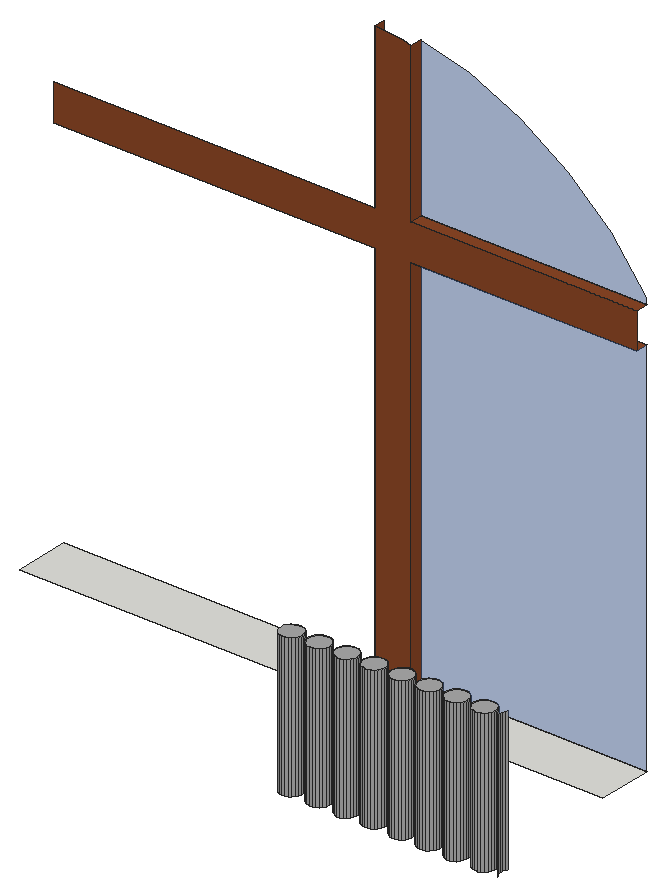
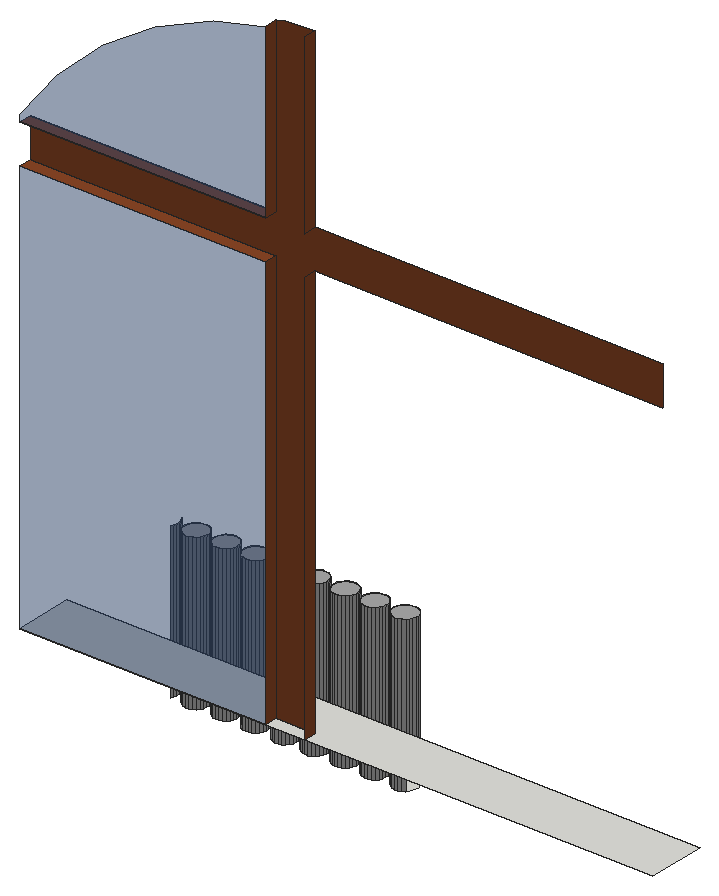
# SketchUp Ruby script. Lengths in inches.
U = 1.inch
M = Sketchup.active_model
def pt(a) = Geom::Point3d.new(a.map { |v| v * U })
def face(e, loops, mat)
  f = e.add_face(loops[0].map { |a| pt(a) })
  loops[1..].each { |l| e.add_face(l.map { |a| pt(a) }).erase! }
  f.material = f.back_material = mat if mat
  f
end
# faces: each face lists its corners as indices into pts; further lists are holes
def faces(e, pts, list, mat = nil) = list.each { |f| face(e, (f[0].is_a?(Array) ? f : [f]).map { |l| l.map { |i| pts[i] } }, mat) }
# xy, xz, yz: faces in a plane at the given z, y or x. An outline is a flat list of corners, or four numbers for a rectangle; further outlines are holes
def ring(l) = l.size == 4 ? [[l[0], l[1]], [l[2], l[1]], [l[2], l[3]], [l[0], l[3]]] : l.each_slice(2).to_a
def flat(e, list, mat, &to3) = list.each { |f| face(e, (f[0].is_a?(Array) ? f : [f]).map { |l| ring(l).map { |u, v| to3.(u, v) } }, mat) }
def xy(e, z, list, mat = nil) = flat(e, list, mat) { |x, y| [x, y, z] }
def xz(e, y, list, mat = nil) = flat(e, list, mat) { |x, z| [x, y, z] }
def yz(e, x, list, mat = nil) = flat(e, list, mat) { |y, z| [x, y, z] }
def lines(e, pts, list) = list.each { |a, b| e.add_line(pt(pts[a]), pt(pts[b])) }
# prism: a flat outline (further loops are holes) pulled along v
def prism(e, loops, v, mat = nil)
  f = face(e, loops, mat); d = Geom::Vector3d.new(v.map { |x| x * U })
  f.pushpull(f.normal.samedirection?(d) ? d.length : -d.length)
end
def box(e, o, s, mat = nil) = prism(e, [[o, [o[0] + s[0], o[1], o[2]], [o[0] + s[0], o[1] + s[1], o[2]], [o[0], o[1] + s[1], o[2]]]], [0, 0, s[2]], mat)
def at(x, y, z, deg = 0) = Geom::Transformation.translation(pt([x, y, z])) * Geom::Transformation.rotation(ORIGIN, Z_AXIS, deg.degrees)
def axes(o, x, y, z) = Geom::Transformation.new([*x, 0, *y, 0, *z, 0, *pt(o).to_a, 1])
def part(name) = M.definitions.add(name)
# library, detail: a bought-in or finely detailed component or shape, given as its bounding box
def library(name, o, s) = part(name).tap { |d| box(d.entities, o, s) }
def detail(e, o, s) = box(e.add_group.entities, o, s)
def put(e, d, t, mat = nil) = e.add_instance(d, t).tap { |i| i.material = mat if mat }
def group(e, t, mat = nil) = e.add_group.tap { |g| g.transformation = t; g.material = mat if mat }.entities
root = M.entities
M.materials.add("[0042_Sienna]").color = [137, 70, 38]
M.materials.add("[0132_LightGray]").color = [169, 169, 169]
M.materials.add("[Translucent Glass Blue]").color = [66, 99, 158]
M.materials["[Translucent Glass Blue]"].alpha = 0.5
xy(root,336.85,[[302.77,32.1,302.31,32.2,301.89,32.42,301.54,32.73,301.28,33.13,301.13,33.58,301.11,34.05,301.2,34.52,301.42,34.9375,301.73,35.29,302.13,35.55,302.58,35.69,303.05,35.72,303.52,35.62,303.9375,35.41,304.29,35.09,304.55,34.69,304.69,34.24,304.72,33.77,304.62,33.31,304.41,32.89,304.09,32.53,303.69,32.28,303.24,32.13],[307.33,32.1,306.87,32.2,306.45,32.42,306.1,32.73,305.84,33.13,305.69,33.58,305.67,34.05,305.77,34.52,305.98,34.9375,306.3,35.29,306.69,35.55,307.14,35.69,307.62,35.72,308.08,35.62,308.5,35.41,308.85,35.09,309.11,34.69,309.26,34.24,309.28,33.77,309.18,33.31,308.97,32.89,308.65,32.53,308.26,32.28,307.81,32.13],[311.9,32.1,311.43,32.2,311.01,32.42,310.66,32.73,310.4,33.13,310.26,33.58,310.23,34.05,310.33,34.52,310.54,34.9375,310.86,35.29,311.26,35.55,311.71,35.69,312.18,35.72,312.64,35.62,313.0625,35.41,313.42,35.09,313.67,34.69,313.82,34.24,313.84,33.77,313.75,33.31,313.53,32.89,313.22,32.53,312.82,32.28,312.37,32.13],[316.46,32.1,316,32.2,315.57,32.42,315.22,32.73,314.97,33.13,314.82,33.58,314.79,34.05,314.89,34.52,315.11,34.9375,315.42,35.29,315.82,35.55,316.27,35.69,316.74,35.72,317.2,35.62,317.625,35.41,317.98,35.09,318.24,34.69,318.38,34.24,318.41,33.77,318.31,33.31,318.09,32.89,317.78,32.53,317.38,32.28,316.93,32.13],[321.02,32.1,320.56,32.2,320.14,32.42,319.79,32.73,319.53,33.13,319.38,33.58,319.36,34.05,319.45,34.52,319.67,34.9375,319.98,35.29,320.38,35.55,320.83,35.69,321.3,35.72,321.77,35.62,322.1875,35.41,322.54,35.09,322.8,34.69,322.94,34.24,322.97,33.77,322.87,33.31,322.66,32.89,322.34,32.53,321.94,32.28,321.49,32.13],
  [325.58,32.1,325.12,32.2,324.7,32.42,324.35,32.73,324.09,33.13,323.94,33.58,323.92,34.05,324.02,34.52,324.23,34.9375,324.55,35.29,324.94,35.55,325.39,35.69,325.87,35.72,326.33,35.62,326.75,35.41,327.1,35.09,327.36,34.69,327.51,34.24,327.53,33.77,327.43,33.31,327.22,32.89,326.9,32.53,326.51,32.28,326.06,32.13],[330.15,32.1,329.68,32.2,329.26,32.42,328.91,32.73,328.65,33.13,328.51,33.58,328.48,34.05,328.58,34.52,328.79,34.9375,329.11,35.29,329.51,35.55,329.96,35.69,330.43,35.72,330.89,35.62,331.3125,35.41,331.67,35.09,331.92,34.69,332.07,34.24,332.09,33.77,332,33.31,331.78,32.89,331.47,32.53,331.07,32.28,330.62,32.13],[334.71,32.1,334.25,32.2,333.82,32.42,333.47,32.73,333.22,33.13,333.07,33.58,333.04,34.05,333.14,34.52,333.36,34.9375,333.67,35.29,334.07,35.55,334.52,35.69,334.99,35.72,335.45,35.62,335.875,35.41,336.23,35.09,336.49,34.69,336.63,34.24,336.66,33.77,336.56,33.31,336.34,32.89,336.03,32.53,335.63,32.28,335.18,32.13]])
xy(root,348.85,[[252.45,40.6875,349.14,40.6875,349.14,49.6875,311.64,49.6875,311.64,47.6875,305.64,47.6875,305.64,49.6875,252.45,49.6875],[305.64,47.6875,311.64,49.6875]])
xy(root,360.41,[[302.77,32.1,303.24,32.13,303.69,32.28,304.09,32.53,304.41,32.89,304.62,33.31,304.72,33.77,304.69,34.24,304.55,34.69,304.29,35.09,303.9375,35.41,303.52,35.62,303.05,35.72,302.58,35.69,302.13,35.55,301.73,35.29,301.42,34.9375,301.2,34.52,301.11,34.05,301.13,33.58,301.28,33.13,301.54,32.73,301.89,32.42,302.31,32.2],[307.33,32.1,307.81,32.13,308.26,32.28,308.65,32.53,308.97,32.89,309.18,33.31,309.28,33.77,309.26,34.24,309.11,34.69,308.85,35.09,308.5,35.41,308.08,35.62,307.62,35.72,307.14,35.69,306.69,35.55,306.3,35.29,305.98,34.9375,305.77,34.52,305.67,34.05,305.69,33.58,305.84,33.13,306.1,32.73,306.45,32.42,306.87,32.2],[311.9,32.1,312.37,32.13,312.82,32.28,313.22,32.53,313.53,32.89,313.75,33.31,313.84,33.77,313.82,34.24,313.67,34.69,313.42,35.09,313.0625,35.41,312.64,35.62,312.18,35.72,311.71,35.69,311.26,35.55,310.86,35.29,310.54,34.9375,310.33,34.52,310.23,34.05,310.26,33.58,310.4,33.13,310.66,32.73,311.01,32.42,311.43,32.2],[316.46,32.1,316.93,32.13,317.38,32.28,317.78,32.53,318.09,32.89,318.31,33.31,318.41,33.77,318.38,34.24,318.24,34.69,317.98,35.09,317.625,35.41,317.2,35.62,316.74,35.72,316.27,35.69,315.82,35.55,315.42,35.29,315.11,34.9375,314.89,34.52,314.79,34.05,314.82,33.58,314.97,33.13,315.22,32.73,315.57,32.42,316,32.2],[321.02,32.1,321.49,32.13,321.94,32.28,322.34,32.53,322.66,32.89,322.87,33.31,322.97,33.77,322.94,34.24,322.8,34.69,322.54,35.09,322.1875,35.41,321.77,35.62,321.3,35.72,320.83,35.69,320.38,35.55,319.98,35.29,319.67,34.9375,319.45,34.52,319.36,34.05,319.38,33.58,319.53,33.13,319.79,32.73,320.14,32.42,320.56,32.2],
  [325.58,32.1,326.06,32.13,326.51,32.28,326.9,32.53,327.22,32.89,327.43,33.31,327.53,33.77,327.51,34.24,327.36,34.69,327.1,35.09,326.75,35.41,326.33,35.62,325.87,35.72,325.39,35.69,324.94,35.55,324.55,35.29,324.23,34.9375,324.02,34.52,323.92,34.05,323.94,33.58,324.09,33.13,324.35,32.73,324.7,32.42,325.12,32.2],[330.15,32.1,330.62,32.13,331.07,32.28,331.47,32.53,331.78,32.89,332,33.31,332.09,33.77,332.07,34.24,331.92,34.69,331.67,35.09,331.3125,35.41,330.89,35.62,330.43,35.72,329.96,35.69,329.51,35.55,329.11,35.29,328.79,34.9375,328.58,34.52,328.48,34.05,328.51,33.58,328.65,33.13,328.91,32.73,329.26,32.42,329.68,32.2],[334.71,32.1,335.18,32.13,335.63,32.28,336.03,32.53,336.34,32.89,336.56,33.31,336.66,33.77,336.63,34.24,336.49,34.69,336.23,35.09,335.875,35.41,335.45,35.62,334.99,35.72,334.52,35.69,334.07,35.55,333.67,35.29,333.36,34.9375,333.14,34.52,333.04,34.05,333.07,33.58,333.22,33.13,333.47,32.73,333.82,32.42,334.25,32.2]],"[0132_LightGray]")
xy(root,412.18,[[311.64,47.6875,349.14,49.6875]],"[0042_Sienna]")
xy(root,418.18,[[311.64,47.6875,349.14,49.6875]],"[0042_Sienna]")
xz(root,47.6875,[[305.64,348.85,311.64,348.85,311.64,412.18,349.14,412.18,349.14,418.18,311.64,418.18,311.64,444.4,310.32,444.74,305.64,445.13,305.64,418.18,252.45,418.18,252.45,412.18,305.64,412.18]],"[0042_Sienna]")
xz(root,49.6875,[[311.64,348.85,349.14,412.18],[311.64,418.18,349.14,418.18,349.14,419.18,343.31,426.75,336.3,433.26,328.32,438.52,319.58,442.38,311.64,444.4]],"[Translucent Glass Blue]")
yz(root,305.64,[[47.6875,348.85,49.6875,412.18],[47.6875,418.18,49.6875,445.13]],"[0042_Sienna]")
yz(root,311.64,[[47.6875,348.85,49.6875,412.18],[47.6875,418.18,49.6875,444.4]],"[0042_Sienna]")
p = [[302.31,32.2,336.85],[302.77,32.1,336.85],[302.77,32.1,360.41],[302.31,32.2,360.41],[303.24,32.13,336.85],[303.24,32.13,360.41],
  [303.69,32.28,336.85],[303.69,32.28,360.41],[306.87,32.2,336.85],[307.33,32.1,336.85],[307.33,32.1,360.41],[306.87,32.2,360.41],
  [307.81,32.13,336.85],[307.81,32.13,360.41],[308.26,32.28,336.85],[308.26,32.28,360.41],[311.43,32.2,336.85],[311.9,32.1,336.85],
  [311.9,32.1,360.41],[311.43,32.2,360.41],[312.37,32.13,336.85],[312.37,32.13,360.41],[312.82,32.28,336.85],[312.82,32.28,360.41],
  [316,32.2,336.85],[316.46,32.1,336.85],[316.46,32.1,360.41],[316,32.2,360.41],[316.93,32.13,336.85],[316.93,32.13,360.41],
  [317.38,32.28,336.85],[317.38,32.28,360.41],[320.56,32.2,336.85],[321.02,32.1,336.85],[321.02,32.1,360.41],[320.56,32.2,360.41],
  [321.49,32.13,336.85],[321.49,32.13,360.41],[321.94,32.28,336.85],[321.94,32.28,360.41],[325.12,32.2,336.85],[325.58,32.1,336.85],
  [325.58,32.1,360.41],[325.12,32.2,360.41],[326.06,32.13,336.85],[326.06,32.13,360.41],[326.51,32.28,336.85],[326.51,32.28,360.41],
  [329.68,32.2,336.85],[330.15,32.1,336.85],[330.15,32.1,360.41],[329.68,32.2,360.41],[330.62,32.13,336.85],[330.62,32.13,360.41],
  [331.07,32.28,336.85],[331.07,32.28,360.41],[334.25,32.2,336.85],[334.71,32.1,336.85],[334.71,32.1,360.41],[334.25,32.2,360.41],
  [335.18,32.13,336.85],[335.18,32.13,360.41],[335.63,32.28,336.85],[335.63,32.28,360.41],[301.89,32.42,336.85],[301.89,32.42,360.41],
  [306.45,32.42,336.85],[306.45,32.42,360.41],[311.01,32.42,336.85],[311.01,32.42,360.41],[315.57,32.42,336.85],[315.57,32.42,360.41],
  [320.14,32.42,336.85],[320.14,32.42,360.41],[324.7,32.42,336.85],[324.7,32.42,360.41],[329.26,32.42,336.85],[329.26,32.42,360.41],
  [333.82,32.42,336.85],[333.82,32.42,360.41],[304.09,32.53,336.85],[304.09,32.53,360.41],[308.65,32.53,336.85],[308.65,32.53,360.41],
  [313.22,32.53,336.85],[313.22,32.53,360.41],[317.78,32.53,336.85],[317.78,32.53,360.41],[322.34,32.53,336.85],[322.34,32.53,360.41],
  [326.9,32.53,336.85],[326.9,32.53,360.41],[331.47,32.53,336.85],[331.47,32.53,360.41],[336.03,32.53,336.85],[336.03,32.53,360.41],
  [301.54,32.73,336.85],[301.54,32.73,360.41],[306.1,32.73,336.85],[306.1,32.73,360.41],[310.66,32.73,336.85],[310.66,32.73,360.41],
  [315.22,32.73,336.85],[315.22,32.73,360.41],[319.79,32.73,336.85],[319.79,32.73,360.41],[324.35,32.73,336.85],[324.35,32.73,360.41],
  [328.91,32.73,336.85],[328.91,32.73,360.41],[333.47,32.73,336.85],[333.47,32.73,360.41],[304.41,32.89,336.85],[304.41,32.89,360.41],
  [308.97,32.89,336.85],[308.97,32.89,360.41],[313.53,32.89,336.85],[313.53,32.89,360.41],[318.09,32.89,336.85],[318.09,32.89,360.41],
  [322.66,32.89,336.85],[322.66,32.89,360.41],[327.22,32.89,336.85],[327.22,32.89,360.41],[331.78,32.89,336.85],[331.78,32.89,360.41],
  [336.34,32.89,336.85],[336.34,32.89,360.41],[305.84,33.13,336.85],[305.84,33.13,360.41],[310.4,33.13,336.85],[310.4,33.13,360.41],
  [314.97,33.13,336.85],[314.97,33.13,360.41],[319.53,33.13,336.85],[319.53,33.13,360.41],[324.09,33.13,336.85],[324.09,33.13,360.41],
  [328.65,33.13,336.85],[328.65,33.13,360.41],[333.22,33.13,336.85],[333.22,33.13,360.41],[337.78,33.13,336.85],[338.04,32.73,336.85],
  [338.04,32.73,360.41],[337.78,33.13,360.41],[304.62,33.31,336.85],[304.62,33.31,360.41],[309.18,33.31,336.85],[309.18,33.31,360.41],
  [313.75,33.31,336.85],[313.75,33.31,360.41],[318.31,33.31,336.85],[318.31,33.31,360.41],[322.87,33.31,336.85],[322.87,33.31,360.41],
  [327.43,33.31,336.85],[327.43,33.31,360.41],[332,33.31,336.85],[332,33.31,360.41],[336.56,33.31,336.85],[336.56,33.31,360.41],
  [305.69,33.58,336.85],[305.69,33.58,360.41],[310.26,33.58,336.85],[310.26,33.58,360.41],[314.82,33.58,336.85],[314.82,33.58,360.41],
  [319.38,33.58,336.85],[319.38,33.58,360.41],[323.94,33.58,336.85],[323.94,33.58,360.41],[328.51,33.58,336.85],[328.51,33.58,360.41],
  [333.07,33.58,336.85],[333.07,33.58,360.41],[337.63,33.58,336.85],[337.63,33.58,360.41],[304.72,33.77,336.85],[304.72,33.77,360.41],
  [309.28,33.77,336.85],[309.28,33.77,360.41],[313.84,33.77,336.85],[313.84,33.77,360.41],[318.41,33.77,336.85],[318.41,33.77,360.41],
  [322.97,33.77,336.85],[322.97,33.77,360.41],[327.53,33.77,336.85],[327.53,33.77,360.41],[332.09,33.77,336.85],[332.09,33.77,360.41],
  [336.66,33.77,336.85],[336.66,33.77,360.41],[305.67,34.05,336.85],[305.67,34.05,360.41],[310.23,34.05,336.85],[310.23,34.05,360.41],
  [314.79,34.05,336.85],[314.79,34.05,360.41],[319.36,34.05,336.85],[319.36,34.05,360.41],[323.92,34.05,336.85],[323.92,34.05,360.41],
  [328.48,34.05,336.85],[328.48,34.05,360.41],[333.04,34.05,336.85],[333.04,34.05,360.41],[337.61,34.05,336.85],[337.61,34.05,360.41],
  [304.69,34.24,336.85],[304.69,34.24,360.41],[309.26,34.24,336.85],[309.26,34.24,360.41],[313.82,34.24,336.85],[313.82,34.24,360.41],
  [318.38,34.24,336.85],[318.38,34.24,360.41],[322.94,34.24,336.85],[322.94,34.24,360.41],[327.51,34.24,336.85],[327.51,34.24,360.41],
  [332.07,34.24,336.85],[332.07,34.24,360.41],[336.63,34.24,336.85],[336.63,34.24,360.41],[305.77,34.52,336.85],[305.77,34.52,360.41],
  [310.33,34.52,336.85],[310.33,34.52,360.41],[314.89,34.52,336.85],[314.89,34.52,360.41],[319.45,34.52,336.85],[319.45,34.52,360.41],
  [324.02,34.52,336.85],[324.02,34.52,360.41],[328.58,34.52,336.85],[328.58,34.52,360.41],[333.14,34.52,336.85],[333.14,34.52,360.41],
  [337.7,34.52,336.85],[337.7,34.52,360.41],[304.55,34.69,336.85],[304.55,34.69,360.41],[309.11,34.69,336.85],[309.11,34.69,360.41],
  [313.67,34.69,336.85],[313.67,34.69,360.41],[318.24,34.69,336.85],[318.24,34.69,360.41],[322.8,34.69,336.85],[322.8,34.69,360.41],
  [327.36,34.69,336.85],[327.36,34.69,360.41],[331.92,34.69,336.85],[331.92,34.69,360.41],[336.49,34.69,336.85],[336.49,34.69,360.41],
  [305.98,34.9375,336.85],[305.98,34.9375,360.41],[310.54,34.9375,336.85],[310.54,34.9375,360.41],[315.11,34.9375,336.85],[315.11,34.9375,360.41],
  [319.67,34.9375,336.85],[319.67,34.9375,360.41],[324.23,34.9375,336.85],[324.23,34.9375,360.41],[328.79,34.9375,336.85],[328.79,34.9375,360.41],
  [333.36,34.9375,336.85],[333.36,34.9375,360.41],[337.92,34.9375,336.85],[337.92,34.9375,360.41],[304.29,35.09,336.85],[304.29,35.09,360.41],
  [308.85,35.09,336.85],[308.85,35.09,360.41],[313.42,35.09,336.85],[313.42,35.09,360.41],[317.98,35.09,336.85],[317.98,35.09,360.41],
  [322.54,35.09,336.85],[322.54,35.09,360.41],[327.1,35.09,336.85],[327.1,35.09,360.41],[331.67,35.09,336.85],[331.67,35.09,360.41],
  [336.23,35.09,336.85],[336.23,35.09,360.41],[306.3,35.29,336.85],[306.3,35.29,360.41],[310.86,35.29,336.85],[310.86,35.29,360.41],
  [315.42,35.29,336.85],[315.42,35.29,360.41],[319.98,35.29,336.85],[319.98,35.29,360.41],[324.55,35.29,336.85],[324.55,35.29,360.41],
  [329.11,35.29,336.85],[329.11,35.29,360.41],[333.67,35.29,336.85],[333.67,35.29,360.41],[303.9375,35.41,336.85],[303.9375,35.41,360.41],
  [308.5,35.41,336.85],[308.5,35.41,360.41],[313.0625,35.41,336.85],[313.0625,35.41,360.41],[317.625,35.41,336.85],[317.625,35.41,360.41],
  [322.1875,35.41,336.85],[322.1875,35.41,360.41],[326.75,35.41,336.85],[326.75,35.41,360.41],[331.3125,35.41,336.85],[331.3125,35.41,360.41],
  [335.875,35.41,336.85],[335.875,35.41,360.41],[302.13,35.55,336.85],[301.73,35.29,336.85],[301.73,35.29,360.41],[302.13,35.55,360.41],
  [306.69,35.55,336.85],[306.69,35.55,360.41],[311.26,35.55,336.85],[311.26,35.55,360.41],[315.82,35.55,336.85],[315.82,35.55,360.41],
  [320.38,35.55,336.85],[320.38,35.55,360.41],[324.94,35.55,336.85],[324.94,35.55,360.41],[329.51,35.55,336.85],[329.51,35.55,360.41],
  [334.07,35.55,336.85],[334.07,35.55,360.41],[303.52,35.62,336.85],[303.52,35.62,360.41],[308.08,35.62,336.85],[308.08,35.62,360.41],
  [312.64,35.62,336.85],[312.64,35.62,360.41],[317.2,35.62,336.85],[317.2,35.62,360.41],[321.77,35.62,336.85],[321.77,35.62,360.41],
  [326.33,35.62,336.85],[326.33,35.62,360.41],[330.89,35.62,336.85],[330.89,35.62,360.41],[335.45,35.62,336.85],[335.45,35.62,360.41],
  [302.58,35.69,336.85],[302.58,35.69,360.41],[307.14,35.69,336.85],[307.14,35.69,360.41],[311.71,35.69,336.85],[311.71,35.69,360.41],
  [316.27,35.69,336.85],[316.27,35.69,360.41],[320.83,35.69,336.85],[320.83,35.69,360.41],[325.39,35.69,336.85],[325.39,35.69,360.41],
  [329.96,35.69,336.85],[329.96,35.69,360.41],[334.52,35.69,336.85],[334.52,35.69,360.41],[303.05,35.72,336.85],[303.05,35.72,360.41],
  [307.62,35.72,336.85],[307.62,35.72,360.41],[312.18,35.72,336.85],[312.18,35.72,360.41],[316.74,35.72,336.85],[316.74,35.72,360.41],
  [321.3,35.72,336.85],[321.3,35.72,360.41],[325.87,35.72,336.85],[325.87,35.72,360.41],[330.43,35.72,336.85],[330.43,35.72,360.41],
  [334.99,35.72,336.85],[334.99,35.72,360.41]]
faces(root,p,[[0,1,2,3],[1,4,5,2],[4,6,7,5],[8,9,10,11],[9,12,13,10],[12,14,15,13],[16,17,18,19],[17,20,21,18],
  [20,22,23,21],[24,25,26,27],[25,28,29,26],[28,30,31,29],[32,33,34,35],[33,36,37,34],[36,38,39,37],[40,41,42,43],
  [41,44,45,42],[44,46,47,45],[48,49,50,51],[49,52,53,50],[52,54,55,53],[56,57,58,59],[57,60,61,58],[60,62,63,61],
  [64,0,3,65],[66,8,11,67],[68,16,19,69],[70,24,27,71],[72,32,35,73],[74,40,43,75],[76,48,51,77],[78,56,59,79],
  [6,80,81,7],[14,82,83,15],[22,84,85,23],[30,86,87,31],[38,88,89,39],[46,90,91,47],[54,92,93,55],[62,94,95,63],
  [96,64,65,97],[98,66,67,99],[100,68,69,101],[102,70,71,103],[104,72,73,105],[106,74,75,107],[108,76,77,109],[110,78,79,111],
  [80,112,113,81],[82,114,115,83],[84,116,117,85],[86,118,119,87],[88,120,121,89],[90,122,123,91],[92,124,125,93],[94,126,127,95],
  [128,98,99,129],[130,100,101,131],[132,102,103,133],[134,104,105,135],[136,106,107,137],[138,108,109,139],[140,110,111,141],[142,143,144,145],
  [112,146,147,113],[114,148,149,115],[116,150,151,117],[118,152,153,119],[120,154,155,121],[122,156,157,123],[124,158,159,125],[126,160,161,127],
  [162,128,129,163],[164,130,131,165],[166,132,133,167],[168,134,135,169],[170,136,137,171],[172,138,139,173],[174,140,141,175],[176,142,145,177],
  [146,178,179,147],[148,180,181,149],[150,182,183,151],[152,184,185,153],[154,186,187,155],[156,188,189,157],[158,190,191,159],[160,192,193,161],
  [194,162,163,195],[196,164,165,197],[198,166,167,199],[200,168,169,201],[202,170,171,203],[204,172,173,205],[206,174,175,207],[208,176,177,209],
  [178,210,211,179],[180,212,213,181],[182,214,215,183],[184,216,217,185],[186,218,219,187],[188,220,221,189],[190,222,223,191],[192,224,225,193],
  [226,194,195,227],[228,196,197,229],[230,198,199,231],[232,200,201,233],[234,202,203,235],[236,204,205,237],[238,206,207,239],[240,208,209,241],
  [210,242,243,211],[212,244,245,213],[214,246,247,215],[216,248,249,217],[218,250,251,219],[220,252,253,221],[222,254,255,223],[224,256,257,225],
  [258,226,227,259],[260,228,229,261],[262,230,231,263],[264,232,233,265],[266,234,235,267],[268,236,237,269],[270,238,239,271],[272,240,241,273],
  [242,274,275,243],[244,276,277,245],[246,278,279,247],[248,280,281,249],[250,282,283,251],[252,284,285,253],[254,286,287,255],[256,288,289,257],
  [290,258,259,291],[292,260,261,293],[294,262,263,295],[296,264,265,297],[298,266,267,299],[300,268,269,301],[302,270,271,303],[274,304,305,275],
  [276,306,307,277],[278,308,309,279],[280,310,311,281],[282,312,313,283],[284,314,315,285],[286,316,317,287],[288,318,319,289],[320,321,322,323],
  [324,290,291,325],[326,292,293,327],[328,294,295,329],[330,296,297,331],[332,298,299,333],[334,300,301,335],[336,302,303,337],[304,338,339,305],
  [306,340,341,307],[308,342,343,309],[310,344,345,311],[312,346,347,313],[314,348,349,315],[316,350,351,317],[318,352,353,319],[354,320,323,355],
  [356,324,325,357],[358,326,327,359],[360,328,329,361],[362,330,331,363],[364,332,333,365],[366,334,335,367],[368,336,337,369],[338,370,371,339],
  [340,372,373,341],[342,374,375,343],[344,376,377,345],[346,378,379,347],[348,380,381,349],[350,382,383,351],[352,384,385,353],[370,354,355,371],
  [372,356,357,373],[374,358,359,375],[376,360,361,377],[378,362,363,379],[380,364,365,381],[382,366,367,383],[384,368,369,385]],"[0132_LightGray]")
